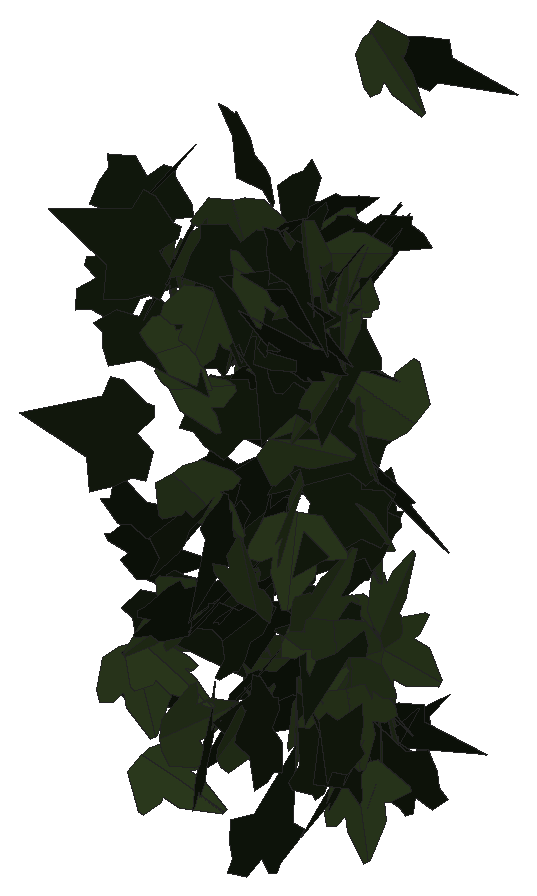
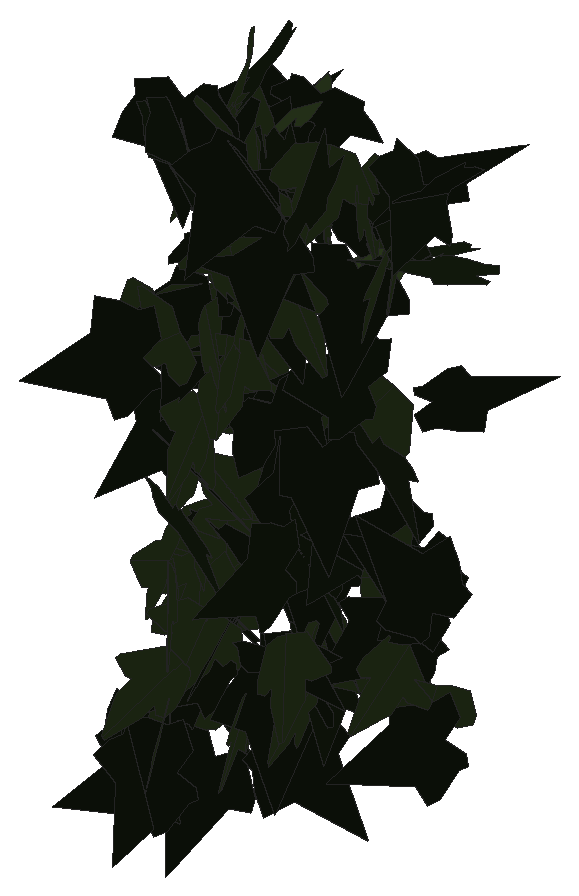
# SketchUp Ruby script. Lengths in inches.
U = 1.inch
M = Sketchup.active_model
def pt(a) = Geom::Point3d.new(a.map { |v| v * U })
def face(e, loops, mat)
  f = e.add_face(loops[0].map { |a| pt(a) })
  loops[1..].each { |l| e.add_face(l.map { |a| pt(a) }).erase! }
  f.material = f.back_material = mat if mat
  f
end
# faces: each face lists its corners as indices into pts; further lists are holes
def faces(e, pts, list, mat = nil) = list.each { |f| face(e, (f[0].is_a?(Array) ? f : [f]).map { |l| l.map { |i| pts[i] } }, mat) }
# xy, xz, yz: faces in a plane at the given z, y or x. An outline is a flat list of corners, or four numbers for a rectangle; further outlines are holes
def ring(l) = l.size == 4 ? [[l[0], l[1]], [l[2], l[1]], [l[2], l[3]], [l[0], l[3]]] : l.each_slice(2).to_a
def flat(e, list, mat, &to3) = list.each { |f| face(e, (f[0].is_a?(Array) ? f : [f]).map { |l| ring(l).map { |u, v| to3.(u, v) } }, mat) }
def xy(e, z, list, mat = nil) = flat(e, list, mat) { |x, y| [x, y, z] }
def xz(e, y, list, mat = nil) = flat(e, list, mat) { |x, z| [x, y, z] }
def yz(e, x, list, mat = nil) = flat(e, list, mat) { |y, z| [x, y, z] }
def lines(e, pts, list) = list.each { |a, b| e.add_line(pt(pts[a]), pt(pts[b])) }
# prism: a flat outline (further loops are holes) pulled along v
def prism(e, loops, v, mat = nil)
  f = face(e, loops, mat); d = Geom::Vector3d.new(v.map { |x| x * U })
  f.pushpull(f.normal.samedirection?(d) ? d.length : -d.length)
end
def box(e, o, s, mat = nil) = prism(e, [[o, [o[0] + s[0], o[1], o[2]], [o[0] + s[0], o[1] + s[1], o[2]], [o[0], o[1] + s[1], o[2]]]], [0, 0, s[2]], mat)
def at(x, y, z, deg = 0) = Geom::Transformation.translation(pt([x, y, z])) * Geom::Transformation.rotation(ORIGIN, Z_AXIS, deg.degrees)
def axes(o, x, y, z) = Geom::Transformation.new([*x, 0, *y, 0, *z, 0, *pt(o).to_a, 1])
def part(name) = M.definitions.add(name)
# library, detail: a bought-in or finely detailed component or shape, given as its bounding box
def library(name, o, s) = part(name).tap { |d| box(d.entities, o, s) }
def detail(e, o, s) = box(e.add_group.entities, o, s)
def put(e, d, t, mat = nil) = e.add_instance(d, t).tap { |i| i.material = mat if mat }
def group(e, t, mat = nil) = e.add_group.tap { |g| g.transformation = t; g.material = mat if mat }.entities
root = M.entities
M.materials.add("efeu1").color = [18, 25, 13]
M.materials.add("efeu2").color = [43, 57, 29]
c1 = part("ivyleaf_10")
p = [[0,0.5,-0.03],[-0.0625,2.02,-0.43],[-0.19,2.01,-0.46],[-0.54,1.05,-0.29],[-0.52,0.625,-0.18],[-0.83,0.76,-0.28],
  [-1.16,0.64,-0.33],[-1.15,0.33,-0.24],[-0.77,-0.39,0.02],[-0.3,-0.51,0.16],[0.04,-0.48,0.23],[-0.02,2.01,-0.4375],
  [-0.06,2.01,-0.43],[0.04,-0.49,0.23],[0.67,-0.49,0.14],[1.38,0.36,-0.2],[1.375,0.51,-0.24],[0.81,0.65,-0.19],
  [0.62,0.59,-0.15],[0.6,1.09,-0.28],[0.5,1.23,-0.31]]
faces(c1.entities,p,[[0,1,2,3,4,5,6,7,8,9,10],[11,12,0,13,14,15,16,17,18,19,20]],"efeu2")
c2 = part("ivyleaf_9")
p = [[1.54,2.16,1.25],[1.36,2.04,1.19],[-0.21,0.99,0.68],[-0.71,1.11,0.82],[-0.85,0.86,0.67],[-0.8,0.17,0.21],
  [-0.9,-0.01,0.1],[-0.67,-0.16,-0.02],[-0.08,-0.08,-0.05],[-0.03,-0.6,-0.4],[0.65,-0.88,-0.66],[0.83,-0.6,-0.49],
  [1.29,-0.42,-0.43],[1.8125,-0.07,-0.26],[1.21,0.44,0.15]]
faces(c2.entities,p,[[0,1,2,3,4,5,6,7,8,9,10,11,12,13,14]],"efeu1")
put(root,c1,axes([51.79,221.74,236.87],[-0.48977,0.09922,0.01674],[0.01457,-0.01236,0.49963],[0.09956,0.4899,0.00921]))
put(root,c2,axes([52.02,222.11,240.14],[-0.03552,-0.39833,0.30011],[0.0501,-0.3022,-0.39518],[0.49621,0.002,0.06138]))
put(root,c2,axes([49.61,222.04,238.39],[-0.16361,-0.33773,-0.33041],[-0.12996,-0.304,0.37509],[-0.45425,0.20862,0.0117]))
put(root,c2,axes([52.625,222.06,240.4],[-0.49314,-0.07283,0.03887],[0.08191,-0.46115,0.17501],[0.01036,0.17897,0.46676]))
put(root,c2,axes([49.98,222.04,241.21],[-0.19844,-0.38743,-0.246],[-0.10675,-0.2217,0.43526],[-0.44635,0.22527,0.00527]))
put(root,c2,axes([51.47,221.93,241.81],[-0.31744,-0.23261,-0.30842],[0.25759,0.17003,-0.39337],[0.28788,-0.40863,0.01189]))
put(root,c2,axes([49.89,221.91,240.2],[0.14281,-0.46905,-0.09796],[0.30059,0.1673,-0.36285],[0.37317,0.04475,0.32976]))
put(root,c1,axes([51.8,221.63,241.625],[0.31572,-0.35482,-0.15629],[0.27593,0.34722,-0.23088],[0.27237,0.05954,0.41506]))
put(root,c2,axes([52.24,222.04,241.9375],[0.22921,-0.43258,0.10165],[0.05429,-0.08627,-0.4895],[0.44104,0.23543,0.00742]))
put(root,c2,axes([52.03,221.6875,233.22],[-0.08028,-0.25566,0.42213],[0.29568,0.3175,0.24853],[-0.39513,0.28953,0.10021]))
put(root,c2,axes([51.08,222.17,237.6],[-0.06978,0.08659,-0.48748],[0.34605,-0.34355,-0.11056],[-0.35409,-0.35281,-0.01198]))
put(root,c2,axes([51.1,221.58,234],[0.04595,0.02864,0.49706],[-0.0328,0.49826,-0.02568],[-0.4968,-0.03025,0.04767]))
put(root,c1,axes([50.79,221.59,239.625],[0.42819,-0.14501,-0.2136],[0.13498,0.47838,-0.05418],[0.22008,-0.01126,0.44882]))
put(root,c2,axes([52,221.87,234.98],[-0.09108,-0.01768,-0.49132],[-0.4861,-0.07152,0.09268],[-0.07355,0.49454,-0.00417]))
put(root,c1,axes([50.22,222.35,235.91],[0.01019,-0.15582,0.47499],[-0.00027,-0.47509,-0.15585],[0.4999,0.00292,-0.00977]))
put(root,c1,axes([50.84,222.02,240.63],[0.49198,0.00602,-0.08901],[-0.0892,0.04218,-0.49017],[0.00161,0.49818,0.04258]))
put(root,c1,axes([52.23,222.09,238.3],[0.24256,-0.43709,-0.01069],[-0.00338,0.01035,-0.49988],[0.43721,0.24257,0.00207]))
put(root,c2,axes([52.14,221.82,241.28],[0.48627,0.11504,0.01743],[0.01768,0.00098,-0.49969],[-0.115,0.48659,-0.00311]))
put(root,c1,axes([50.51,221.67,240.08],[0.42699,-0.09912,-0.24053],[0.13494,0.47962,0.04191],[0.22242,-0.1007,0.43634]))
put(root,c2,axes([52.25,222.34,241.01],[-0.08736,0.03649,0.49096],[-0.37091,-0.33275,-0.04127],[0.32371,-0.37141,0.0852]))
put(root,c2,axes([50.67,221.85,237.42],[-0.22338,0.41974,0.15467],[-0.09613,0.1238,-0.4748],[-0.43688,-0.24185,0.02539]))
put(root,c2,axes([50.27,221.7,236.06],[0.05246,0.39522,-0.30174],[0.01287,0.30223,0.39811],[0.49707,-0.04954,0.02154]))
put(root,c1,axes([50.59,221.97,238.02],[-0.36452,-0.14051,-0.31206],[0.29876,0.09174,-0.39029],[0.16693,-0.471,0.01707]))
put(root,c1,axes([52.37,222.23,242.1],[-0.15022,0.41437,-0.23607],[0.09652,-0.21596,-0.4405],[-0.46703,-0.17792,-0.0151]))
put(root,c1,axes([49.8125,222.24,235.09],[0.01301,-0.49759,0.04733],[0.48981,0.00325,-0.10038],[0.09959,0.04897,0.48753]))
put(root,c1,axes([50.55,221.82,234.41],[0.01643,-0.04538,0.49766],[-0.02406,0.49728,0.04614],[-0.49915,-0.02546,0.01416]))
put(root,c2,axes([51.2,222.09,240.47],[-0.3645,0.01905,-0.34173],[-0.34116,-0.0602,0.36053],[-0.02741,0.496,0.05688]))
put(root,c2,axes([51.83,222.13,241.12],[-0.2461,0.43237,-0.0499],[0.02673,-0.0422,-0.4975],[-0.43442,-0.24753,-0.00235]))
put(root,c1,axes([49.89,222.24,233.49],[0.01263,-0.48309,-0.12831],[0.48888,0.03866,-0.09747],[0.10409,-0.123,0.47333]))
put(root,c1,axes([51.3125,221.96,234.4375],[0.12506,-0.24271,0.41887],[-0.11404,0.40568,0.26911],[-0.47048,-0.16285,0.04611]))
put(root,c1,axes([51.21,222.18,240.59],[0.25728,-0.38075,-0.19707],[-0.05153,0.20071,-0.45504],[0.42562,0.25446,0.06404]))
put(root,c2,axes([50.93,222.12,239.26],[0.37514,-0.29143,-0.15601],[0.18678,0.38157,-0.26366],[0.27273,0.13954,0.39515]))
put(root,c2,axes([50.13,222.45,241.13],[-0.33769,0.18315,-0.32004],[0.24426,-0.21399,-0.38019],[-0.27624,-0.41311,0.05505]))
put(root,c2,axes([51.61,221.97,240.63],[0.49301,-0.05073,-0.06611],[0.02721,0.47294,-0.15997],[0.07876,0.15414,0.46908]))
put(root,c1,axes([52.28,222.42,241.33],[0.01428,-0.49916,0.02515],[0.01048,-0.02486,-0.49927],[0.49969,0.01479,0.00975]))
put(root,c1,axes([52.32,222.73,239.83],[0.02652,-0.22721,0.4446],[0.14274,-0.4232,-0.22479],[0.47846,0.13884,0.04242]))
put(root,c1,axes([50.31,222.5,241.24],[0.14028,-0.47447,0.07208],[0.09684,-0.04557,-0.48841],[0.47005,0.15099,0.07911]))
put(root,c1,axes([51.96,222.43,237.58],[0.40336,0.29443,-0.02469],[-0.01795,-0.01729,-0.49938],[-0.29492,0.40375,-0.00337]))
put(root,c2,axes([49,222.1875,240.39],[0.45456,-0.20366,-0.04358],[0.17617,0.43178,-0.18037],[0.1111,0.14862,0.46429]))
put(root,c2,axes([52.75,222.18,234.52],[-0.01828,0.26912,0.421],[-0.3059,0.32708,-0.22236],[-0.39508,-0.2657,0.15269]))
put(root,c2,axes([51.9,222.3,240.56],[0.24968,-0.26781,-0.34049],[-0.18876,0.28647,-0.36374],[0.38991,0.31018,0.04195]))
put(root,c2,axes([50.91,222.1,236.27],[0.09823,0.38554,0.30284],[0.00356,0.30829,-0.39363],[-0.49024,0.07949,0.05782]))
put(root,c1,axes([52.2,222.37,241.52],[-0.3804,0.12576,0.29913],[-0.28368,0.0949,-0.40065],[-0.15755,-0.47453,-0.00085]))
put(root,c2,axes([51.36,222.25,235.87],[-0.16188,0.35727,0.31009],[-0.16107,0.26654,-0.39117],[-0.44481,-0.22654,0.02879]))
put(root,c2,axes([49.28,222.76,241.66],[-0.04486,-0.49754,-0.02104],[0.04136,0.01733,-0.49799],[0.49626,-0.04642,0.0396]))
put(root,c1,axes([49.29,222.53,234.69],[0.35059,0.33244,0.12874],[0.08332,0.09915,-0.48294],[-0.34662,0.36007,0.01413]))
put(root,c2,axes([52.33,223,234.28],[-0.08945,-0.23726,0.43093],[0.03488,-0.43996,-0.23499],[0.4907,-0.01198,0.09526]))
put(root,c1,axes([49.83,222.47,240.79],[-0.29549,0.38299,0.12653],[-0.10272,0.08022,-0.48271],[-0.39005,-0.31126,0.03127]))
put(root,c2,axes([51.08,222.44,236.1],[0.26205,0.38538,-0.18114],[-0.12231,-0.13562,-0.46546],[-0.40788,0.28826,0.02319]))
put(root,c1,axes([51.71,222.7,240.01],[0.46175,0.17427,-0.08012],[-0.07391,-0.03107,-0.49353],[-0.177,0.46761,-0.00294]))
put(root,c1,axes([51.82,222.43,238.89],[-0.16688,-0.17236,-0.43869],[0.3049,0.31541,-0.23991],[0.35943,-0.34758,-0.00016]))
put(root,c2,axes([49.13,222.66,236.18],[0.35085,0.17601,-0.30971],[0.27646,0.13961,0.39253],[0.22466,-0.44668,0.00065]))
put(root,c1,axes([52.14,222.63,236.33],[-0.02641,-0.44454,0.22734],[0.01246,0.227,0.44532],[-0.49915,0.02919,-0.00091]))
put(root,c2,axes([50.15,222.77,238.74],[0.36467,-0.19099,0.28379],[0.26628,-0.10189,-0.41075],[0.21473,0.45071,0.0274]))
put(root,c1,axes([51.82,222.75,240.71],[0.4447,0.15584,0.16721],[0.15812,0.0544,-0.47121],[-0.16506,0.47197,-0.0009]))
put(root,c1,axes([52.37,222.77,236.11],[-0.41042,-0.28523,0.01417],[-0.0114,-0.00842,-0.4998],[0.28536,-0.41057,0.00041]))
put(root,c2,axes([51.75,222.79,240.08],[-0.185,0.41966,-0.19915],[0.07128,-0.18618,-0.45854],[-0.45902,-0.19805,0.00906]))
put(root,c2,axes([51.5625,222.78,239.88],[0.04768,0.42669,-0.25625],[-0.05269,-0.25165,-0.42883],[-0.49492,0.0679,0.02096]))
put(root,c2,axes([52.12,223.02,236.17],[-0.40116,-0.17128,-0.24441],[0.24238,0.05195,-0.43423],[0.17414,-0.46687,0.04134]))
put(root,c2,axes([52.55,222.89,234.26],[-0.35109,0.31816,-0.15973],[0.12647,-0.09824,-0.47366],[-0.33278,-0.373,-0.01149]))
put(root,c1,axes([52.12,222.87,236.08],[0.38077,0.32306,0.02536],[0.01915,0.01664,-0.49936],[-0.32349,0.38125,0.0003]))
put(root,c2,axes([51.08,222.47,236.24],[0.20119,0.35495,0.28902],[0.06263,0.29139,-0.40146],[-0.45343,0.19775,0.07279]))
put(root,c2,axes([52.08,223.09,240.27],[-0.17123,-0.46061,-0.09228],[0.02934,0.08754,-0.4914],[0.46885,-0.1737,-0.00296]))
put(root,c2,axes([50.3,222.72,240.18],[0.23765,0.41548,-0.14459],[-0.05971,-0.13235,-0.47845],[-0.43584,0.24467,-0.01329]))
put(root,c2,axes([51.3125,223.01,238.12],[-0.04198,0.315,-0.38602],[0.01487,-0.38642,-0.31695],[-0.49801,-0.03809,0.02307]))
put(root,c2,axes([49.62,222.76,235.65],[-0.06086,-0.09484,-0.48714],[0.26498,0.40876,-0.11269],[0.41962,-0.27188,0.0005]))
put(root,c1,axes([52.47,222.93,235.04],[-0.34737,-0.35551,-0.05429],[0.09875,-0.02171,-0.48967],[0.34581,-0.35092,0.0853]))
put(root,c2,axes([49.03,222.73,234.3],[0.43497,0.07511,0.23485],[0.23394,0.02477,-0.4412],[-0.07791,0.4937,-0.0136]))
put(root,c2,axes([49.45,222.56,241.58],[0.046,0.41858,0.26959],[-0.01274,0.27163,-0.41959],[-0.49772,0.03173,0.03565]))
put(root,c2,axes([50.88,222.64,234.68],[-0.06088,0.45849,0.18996],[-0.05168,0.18449,-0.46184],[-0.49358,-0.07587,0.02493]))
put(root,c1,axes([49.83,222.8125,240.52],[-0.24635,0.42276,0.1029],[-0.04951,0.09024,-0.48929],[-0.43227,-0.25126,-0.0026]))
put(root,c1,axes([52.39,223.1,241.08],[-0.07138,0.43316,-0.23933],[-0.00263,-0.24213,-0.43745],[-0.49487,-0.06119,0.03684]))
put(root,c2,axes([48.93,223.06,236.28],[0.00742,-0.101,0.48964],[0.42633,-0.2545,-0.05895],[0.26113,0.41837,0.08234]))
put(root,c1,axes([50.64,222.93,241.6],[-0.45931,-0.18452,-0.07063],[0.06415,0.02977,-0.49497],[0.18687,-0.46375,-0.00367]))
put(root,c1,axes([52.13,223.07,241.48],[0.15006,-0.09276,-0.46784],[0.44866,-0.13894,0.17146],[-0.16182,-0.47126,0.04154]))
put(root,c2,axes([52.24,223.38,237.86],[-0.29221,-0.37476,0.15546],[-0.03934,-0.16452,-0.47052],[0.40381,-0.28721,0.06667]))
put(root,c1,axes([52.5,222.98,235.59],[-0.48911,-0.06005,0.08465],[-0.08528,0.00011,-0.49267],[0.05915,-0.49638,-0.01035]))
put(root,c1,axes([49.5,222.91,235.27],[-0.14635,-0.33149,-0.34452],[0.17221,0.29956,-0.36139],[0.44601,-0.22444,0.02649]))
put(root,c2,axes([50.57,223.03,237.79],[0.26563,0.32031,-0.27721],[-0.20267,-0.19122,-0.41516],[-0.37197,0.33292,0.02825]))
put(root,c1,axes([50.96,223.15,239.83],[-0.39117,0.05506,0.30652],[-0.31143,-0.06856,-0.38511],[-0.00038,-0.49221,0.08793]))
put(root,c1,axes([52.44,223.2,241.46],[0.24375,-0.42753,-0.08836],[-0.05061,0.07284,-0.49207],[0.43362,0.24883,-0.00776]))
put(root,c1,axes([52.625,223,239.03],[-0.32243,0.28652,0.25287],[-0.20373,0.15103,-0.43091],[-0.32331,-0.38091,0.01935]))
put(root,c1,axes([51.3,223.375,234.5],[-0.21714,0.35899,-0.27199],[0.04376,-0.2837,-0.40939],[-0.44826,-0.20159,0.09179]))
put(root,c1,axes([52.41,223.1875,233.69],[0.18261,0.46494,0.02195],[0.00733,0.0207,-0.49952],[-0.4654,0.18276,0.00075]))
put(root,c2,axes([52.1,223.6,238.68],[-0.43968,-0.19164,0.14126],[-0.11627,-0.08603,-0.47862],[0.20775,-0.45373,0.03108]))
put(root,c2,axes([52.75,223.24,241.58],[-0.27604,0.41677,0.01017],[-0.00485,0.00899,-0.4999],[-0.41687,-0.27608,-0.00092]))
put(root,c2,axes([52.52,223.23,241.92],[0.2475,0.37189,-0.22459],[-0.13265,-0.18145,-0.44663],[-0.4137,0.28066,0.00884]))
put(root,c1,axes([51.4,223.62,239.12],[-0.08407,0.38927,-0.30233],[-0.06069,-0.31254,-0.38553],[-0.48913,-0.02812,0.0998]))
put(root,c2,axes([52.5,223.28,241.69],[-0.16299,0.47247,0.01424],[-0.00368,0.0138,-0.4998],[-0.47267,-0.16303,-0.00102]))
put(root,c2,axes([51.33,223.5625,241.6875],[-0.4699,0.12358,-0.11799],[0.1177,-0.01618,-0.48568],[-0.12386,-0.48422,-0.01389]))
put(root,c1,axes([52.25,223.39,237.51],[-0.46906,0.1705,-0.0302],[0.03244,0.00085,-0.49895],[-0.17008,-0.47003,-0.01186]))
put(root,c2,axes([50.61,223.58,234.04],[-0.13103,0.33316,-0.34905],[-0.03436,-0.36722,-0.33759],[-0.4813,-0.06448,0.11913]))
put(root,c1,axes([52.68,223.65,239.08],[0.21372,0.22024,0.39474],[-0.27314,-0.28498,0.30689],[0.36017,-0.34681,-0.0015]))
put(root,c2,axes([52.46,223.63,237.51],[-0.48129,0.13524,-0.00825],[0.00009,-0.03012,-0.49909],[-0.13549,-0.48042,0.02897]))
put(root,c2,axes([50.93,223.25,236.99],[0.02559,-0.0018,0.49934],[0.11616,0.4863,-0.0042],[-0.48565,0.11622,0.02531]))
put(root,c1,axes([51.42,223.64,240.47],[0.41773,0.26972,-0.05248],[-0.04012,-0.03461,-0.49718],[-0.27184,0.41959,-0.00727]))
put(root,c2,axes([51.13,223.47,240.74],[0.31469,0.28574,-0.26329],[-0.20321,-0.16775,-0.42493],[-0.33117,0.37445,0.01055]))
put(root,c2,axes([50.86,223.47,234.67],[0.15045,0.46077,-0.1227],[-0.04146,-0.11553,-0.4847],[-0.47502,0.15602,0.00345]))
put(root,c1,axes([51.67,223.73,239.41],[0.12954,-0.48119,-0.04091],[-0.01606,0.03804,-0.49829],[0.48266,0.13041,-0.0056]))
put(root,c2,axes([51.94,223.45,239.48],[0.39156,0.29379,-0.10185],[-0.11671,-0.01294,-0.48602],[-0.28821,0.40438,0.05844]))
put(root,c1,axes([51.55,223.71,239.05],[-0.48742,-0.1085,0.02555],[-0.02324,-0.01318,-0.49929],[0.10901,-0.48791,0.00781]))
put(root,c1,axes([50.35,223.5625,235.52],[-0.30111,0.35359,0.18521],[-0.10849,0.15077,-0.46422],[-0.38414,-0.31975,-0.01407]))
put(root,c2,axes([49.93,224.13,241.67],[-0.08436,-0.20095,0.45],[0.1046,-0.45345,-0.18288],[0.4816,0.06329,0.11854]))
put(root,c1,axes([51.19,223.66,234.37],[0.11331,-0.44609,-0.19536],[0.13488,0.22147,-0.4275],[0.46794,0.04418,0.17053]))
put(root,c2,axes([51.35,223.52,241.5],[0.25991,0.41547,0.09917],[0.05705,0.08128,-0.49004],[-0.42331,0.26605,-0.00516]))
put(root,c2,axes([51.64,223.93,234.84],[0.03305,-0.46215,0.18796],[0.03073,0.18989,0.46151],[-0.49796,-0.01895,0.04095]))
put(root,c2,axes([52.22,223.74,237.97],[0.49434,-0.07178,-0.02174],[-0.02113,0.00577,-0.49952],[0.07197,0.49479,0.00267]))
put(root,c1,axes([50.48,223.5,234.74],[-0.00161,0.20898,0.45423],[-0.19534,0.41787,-0.19294],[-0.46026,-0.17807,0.0803]))
put(root,c2,axes([51.52,223.81,235.06],[0.47691,-0.1416,0.05002],[0.04649,-0.01916,-0.49747],[0.1428,0.47915,-0.00511]))
put(root,c1,axes([52.32,223.69,233.77],[0.11931,-0.29093,-0.38875],[-0.15229,0.35769,-0.31443],[0.46106,0.19343,-0.00326]))
put(root,c2,axes([52.62,224.02,233.3],[0.15069,-0.12712,0.45949],[-0.37555,0.26521,0.19653],[-0.29369,-0.40436,-0.01555]))
put(root,c2,axes([52.17,223.82,236.78],[-0.25436,0.36473,0.22863],[-0.14612,0.17664,-0.44435],[-0.40491,-0.29287,0.01673]))
put(root,c1,axes([52.43,223.67,235.96],[-0.00707,0.22021,-0.44884],[0.00895,0.44887,0.22008],[0.49987,-0.00492,-0.01029]))
put(root,c1,axes([51.56,224.01,235.52],[0.43312,0.15601,0.1951],[0.13836,0.17531,-0.44735],[-0.20799,0.4415,0.10869]))
put(root,c2,axes([51.47,223.99,233.73],[0.37443,0.31826,-0.09225],[-0.08383,-0.04369,-0.49098],[-0.32058,0.38315,0.02065]))
put(root,c1,axes([51.78,223.91,238.15],[0.03563,0.27982,0.41283],[-0.21374,0.38252,-0.24083],[-0.45061,-0.15932,0.14687]))
put(root,c1,axes([51.94,224.16,236.03],[0.28088,-0.37531,-0.17392],[0.00274,0.21191,-0.45287],[0.41364,0.25345,0.1211]))
put(root,c2,axes([50.14,224.57,235.97],[-0.44577,-0.22633,0.00771],[-0.01093,0.00448,-0.49986],[0.2262,-0.44582,-0.00894]))
put(root,c1,axes([52.02,224.28,234.26],[-0.31542,0.38776,0.0125],[-0.02843,-0.00704,-0.49914],[-0.38691,-0.31559,0.02649]))
put(root,c1,axes([51.85,224.41,234.9375],[0.0948,0.28708,0.39825],[0.07491,0.3924,-0.30069],[-0.48518,0.11668,0.03139]))
put(root,c2,axes([51.65,224.53,233.74],[0.404,0.08371,0.28245],[0.27489,0.06529,-0.41252],[-0.10594,0.4886,0.00673]))
put(root,c2,axes([51.95,224.47,233.6875],[0.10671,0.44511,0.20122],[0.0338,0.19875,-0.45756],[-0.48731,0.11125,0.01233]))
put(root,c1,axes([49.36,225.21,236.41],[-0.0598,-0.48354,-0.1123],[0.03324,0.10896,-0.48685],[0.4953,-0.06569,0.01912]))
put(root,c2,axes([49.41,225.27,237.58],[0.46036,-0.17684,0.08244],[0.08267,-0.01458,-0.4929],[0.17673,0.46746,0.01581]))
put(root,c1,axes([49.43,227.31,241.64],[0.28274,-0.03204,0.41113],[0.41109,0.06126,-0.27794],[-0.03256,0.4952,0.06098]))
put(root,c2,axes([49.65,227.67,241.4375],[0.40512,0.02554,0.29194],[0.29107,0.02277,-0.40591],[-0.03403,0.49883,0.00358]))
